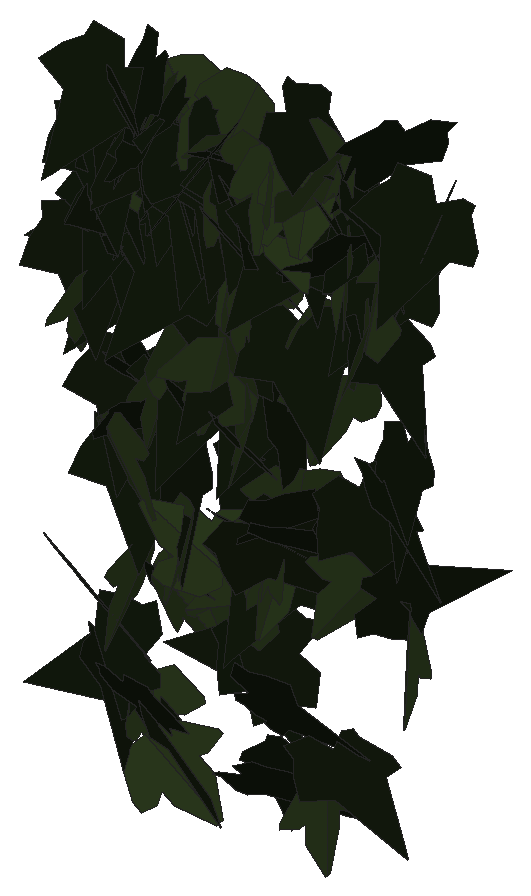
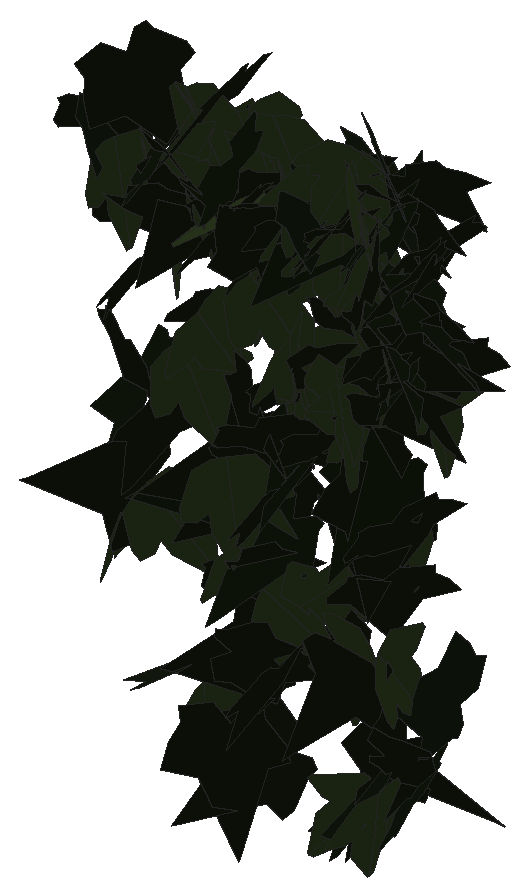
# SketchUp Ruby script. Lengths in inches.
U = 1.inch
M = Sketchup.active_model
def pt(a) = Geom::Point3d.new(a.map { |v| v * U })
def face(e, loops, mat)
  f = e.add_face(loops[0].map { |a| pt(a) })
  loops[1..].each { |l| e.add_face(l.map { |a| pt(a) }).erase! }
  f.material = f.back_material = mat if mat
  f
end
# faces: each face lists its corners as indices into pts; further lists are holes
def faces(e, pts, list, mat = nil) = list.each { |f| face(e, (f[0].is_a?(Array) ? f : [f]).map { |l| l.map { |i| pts[i] } }, mat) }
# xy, xz, yz: faces in a plane at the given z, y or x. An outline is a flat list of corners, or four numbers for a rectangle; further outlines are holes
def ring(l) = l.size == 4 ? [[l[0], l[1]], [l[2], l[1]], [l[2], l[3]], [l[0], l[3]]] : l.each_slice(2).to_a
def flat(e, list, mat, &to3) = list.each { |f| face(e, (f[0].is_a?(Array) ? f : [f]).map { |l| ring(l).map { |u, v| to3.(u, v) } }, mat) }
def xy(e, z, list, mat = nil) = flat(e, list, mat) { |x, y| [x, y, z] }
def xz(e, y, list, mat = nil) = flat(e, list, mat) { |x, z| [x, y, z] }
def yz(e, x, list, mat = nil) = flat(e, list, mat) { |y, z| [x, y, z] }
def lines(e, pts, list) = list.each { |a, b| e.add_line(pt(pts[a]), pt(pts[b])) }
# prism: a flat outline (further loops are holes) pulled along v
def prism(e, loops, v, mat = nil)
  f = face(e, loops, mat); d = Geom::Vector3d.new(v.map { |x| x * U })
  f.pushpull(f.normal.samedirection?(d) ? d.length : -d.length)
end
def box(e, o, s, mat = nil) = prism(e, [[o, [o[0] + s[0], o[1], o[2]], [o[0] + s[0], o[1] + s[1], o[2]], [o[0], o[1] + s[1], o[2]]]], [0, 0, s[2]], mat)
def at(x, y, z, deg = 0) = Geom::Transformation.translation(pt([x, y, z])) * Geom::Transformation.rotation(ORIGIN, Z_AXIS, deg.degrees)
def axes(o, x, y, z) = Geom::Transformation.new([*x, 0, *y, 0, *z, 0, *pt(o).to_a, 1])
def part(name) = M.definitions.add(name)
# library, detail: a bought-in or finely detailed component or shape, given as its bounding box
def library(name, o, s) = part(name).tap { |d| box(d.entities, o, s) }
def detail(e, o, s) = box(e.add_group.entities, o, s)
def put(e, d, t, mat = nil) = e.add_instance(d, t).tap { |i| i.material = mat if mat }
def group(e, t, mat = nil) = e.add_group.tap { |g| g.transformation = t; g.material = mat if mat }.entities
root = M.entities
M.materials.add("efeu1").color = [18, 25, 13]
M.materials.add("efeu2").color = [43, 57, 29]
c1 = part("ivyleaf_10")
p = [[0,0.5,-0.03],[-0.0625,2.02,-0.43],[-0.19,2.01,-0.46],[-0.54,1.05,-0.29],[-0.52,0.625,-0.18],[-0.83,0.76,-0.28],
  [-1.16,0.64,-0.33],[-1.15,0.33,-0.24],[-0.77,-0.39,0.02],[-0.3,-0.51,0.16],[0.04,-0.48,0.23],[-0.02,2.01,-0.4375],
  [-0.06,2.01,-0.43],[0.04,-0.49,0.23],[0.67,-0.49,0.14],[1.38,0.36,-0.2],[1.375,0.51,-0.24],[0.81,0.65,-0.19],
  [0.62,0.59,-0.15],[0.6,1.09,-0.28],[0.5,1.23,-0.31]]
faces(c1.entities,p,[[0,1,2,3,4,5,6,7,8,9,10],[11,12,0,13,14,15,16,17,18,19,20]],"efeu2")
c2 = part("ivyleaf_9")
p = [[1.54,2.16,1.25],[1.36,2.04,1.19],[-0.21,0.99,0.68],[-0.71,1.11,0.82],[-0.85,0.86,0.67],[-0.8,0.17,0.21],
  [-0.9,-0.01,0.1],[-0.67,-0.16,-0.02],[-0.08,-0.08,-0.05],[-0.03,-0.6,-0.4],[0.65,-0.88,-0.66],[0.83,-0.6,-0.49],
  [1.29,-0.42,-0.43],[1.8125,-0.07,-0.26],[1.21,0.44,0.15]]
faces(c2.entities,p,[[0,1,2,3,4,5,6,7,8,9,10,11,12,13,14]],"efeu1")
put(root,c1,axes([46.42,222.2,239.09],[-0.18687,-0.45242,0.10196],[0.01066,-0.11409,-0.48669],[0.46364,-0.17973,0.05229]))
put(root,c1,axes([48.57,222.03,240.14],[0.19422,-0.41581,-0.19845],[-0.07159,0.18551,-0.45876],[0.45514,0.20661,0.01252]))
put(root,c1,axes([47.91,222.2,234.14],[-0.01441,-0.49777,0.04491],[0.14775,-0.04716,-0.47534],[0.47745,-0.00043,0.14845]))
put(root,c2,axes([48.07,222.21,234.64],[0.17664,-0.46352,-0.06285],[0.1854,0.13106,-0.44548],[0.42945,0.13407,0.21817]))
put(root,c1,axes([47.25,222.21,241.76],[0.23344,0.42123,-0.13441],[-0.08511,-0.10634,-0.48109],[-0.43389,0.24749,0.02205]))
put(root,c2,axes([47.02,222.09,235.06],[0.41586,-0.08524,0.26419],[0.25869,-0.05361,-0.42451],[0.10069,0.48976,-0.00049]))
put(root,c2,axes([47.41,222.5,240.875],[-0.31856,-0.36533,0.12269],[-0.08262,-0.09074,-0.48471],[0.37642,-0.32909,-0.00255]))
put(root,c2,axes([47.125,221.98,237.26],[-0.04423,-0.06313,-0.49402],[0.1932,0.45496,-0.07543],[0.45904,-0.19756,-0.01585]))
put(root,c2,axes([44.83,222.46,241.98],[-0.41084,-0.28433,0.01913],[-0.00302,-0.02921,-0.49914],[0.28496,-0.41025,0.02228]))
put(root,c1,axes([46.875,222.07,238.46],[0.2035,-0.33058,-0.31513],[-0.16599,0.26787,-0.38819],[0.42548,0.26261,-0.00072]))
put(root,c1,axes([46.9375,222.19,241.64],[0.41646,-0.22108,-0.16639],[-0.12125,0.12446,-0.46884],[0.24872,0.43085,0.05006]))
put(root,c1,axes([45.87,222.27,236.7],[0.34721,-0.35866,-0.02838],[-0.00942,0.03036,-0.49899],[0.35966,0.34704,0.01432]))
put(root,c2,axes([45.65,221.98,241.66],[-0.16626,0.41848,0.21733],[-0.16013,0.16664,-0.44338],[-0.44353,-0.21703,0.07861]))
put(root,c2,axes([45.83,222.42,239.98],[-0.47455,-0.15731,-0.00731],[0.00761,0.00027,-0.49994],[0.15729,-0.47461,0.00214]))
put(root,c1,axes([48.63,222.18,240.17],[0.40084,-0.28958,0.07396],[-0.05901,0.04462,0.4945],[-0.29299,-0.40516,0.0016]))
put(root,c1,axes([44.57,222.27,239.35],[0.0171,-0.49805,-0.04069],[0.00491,0.04088,-0.4983],[0.49968,0.01664,0.00629]))
put(root,c1,axes([44.9,222.29,237.51],[-0.33765,0.2221,-0.29439],[0.25155,-0.15316,-0.40406],[-0.26966,-0.42097,-0.00831]))
put(root,c2,axes([47.24,221.97,237.3],[0.32648,0.13241,0.35479],[0.31842,0.15757,-0.35182],[-0.20498,0.45567,0.01856]))
put(root,c2,axes([46.6,222.63,240.59],[-0.02732,-0.24224,0.43654],[0.10822,-0.42968,-0.23166],[0.48738,0.08183,0.07591]))
put(root,c2,axes([45.21,222.1,234.53],[0.46391,0.06793,-0.17372],[-0.17364,-0.01278,-0.46871],[-0.06812,0.4952,0.01173]))
put(root,c2,axes([44.73,222.68,240.35],[-0.07226,-0.19063,0.45655],[-0.09926,-0.44643,-0.20211],[0.48469,-0.11984,0.02668]))
put(root,c2,axes([48.58,222.43,238.05],[0.29534,-0.38285,0.12727],[0.07739,-0.10104,-0.48353],[0.39596,0.30531,-0.00043]))
put(root,c2,axes([47.3,222.1,237.08],[0.40834,-0.06084,0.28206],[0.28835,0.10414,-0.39498],[-0.01068,0.48524,0.12014]))
put(root,c1,axes([48.93,222.48,236.27],[-0.13278,0.34249,-0.33922],[0.07943,-0.33149,-0.36579],[-0.47546,-0.15103,0.03362]))
put(root,c2,axes([44.22,222.4,235.53],[0.32861,-0.28889,0.24199],[0.19161,-0.14838,-0.43734],[0.3245,0.38016,0.01319]))
put(root,c1,axes([46.89,222.13,240.04],[-0.05069,0.47946,0.13248],[-0.02425,0.13062,-0.48203],[-0.49683,-0.0553,0.01001]))
put(root,c1,axes([46.97,222.31,236.84],[0.4392,-0.19955,-0.13145],[-0.10824,0.07909,-0.4817],[0.21304,0.45158,0.02627]))
put(root,c2,axes([44.55,222.48,241.1875],[0.02173,-0.49573,-0.06147],[0.02959,0.0627,-0.49517],[0.49865,0.01788,0.03207]))
put(root,c2,axes([45.24,222.5,238.07],[0.10524,-0.14329,0.46732],[0.32516,-0.33639,-0.17637],[0.36495,0.34104,0.02238]))
put(root,c1,axes([44.99,222.59,235.8],[0.11629,-0.39728,0.28044],[0.09858,-0.2631,-0.4136],[0.47619,0.15149,0.01714]))
put(root,c1,axes([45.5,222.47,238.5],[0.07603,-0.48302,0.10444],[0.03952,-0.09939,-0.48843],[0.4926,0.08253,0.02307]))
put(root,c2,axes([46.37,222.27,240.68],[0.45637,-0.20428,0.0008],[0.02021,0.04322,-0.49772],[0.20327,0.45432,0.04771]))
put(root,c2,axes([45.48,222.54,241.5],[-0.49125,-0.09,0.02399],[-0.02451,0.00067,-0.4994],[0.08986,-0.49183,-0.00507]))
put(root,c2,axes([47.375,222.48,239.6],[-0.1139,-0.44482,-0.1979],[0.09754,0.17828,-0.45684],[0.47698,-0.14268,0.04616]))
put(root,c2,axes([45.27,222.49,242.21],[-0.37767,0.10785,-0.30942],[0.30192,-0.06892,-0.39254],[-0.12732,-0.48334,-0.01306]))
put(root,c2,axes([45.17,222.73,241.25],[0.00783,-0.37095,0.33517],[0.06732,-0.33137,-0.36832],[0.49539,0.05089,0.04475]))
put(root,c2,axes([44.41,222.51,239.86],[-0.15924,-0.43992,-0.17638],[0.0508,0.16915,-0.46777],[0.47123,-0.16689,-0.00917]))
put(root,c1,axes([46.71,222.22,238.8],[-0.06522,0.04191,-0.49395],[-0.42133,0.25783,0.07751],[0.2612,0.42634,0.00168]))
put(root,c2,axes([46,222.65,240.91],[-0.20325,-0.45671,-0.01015],[-0.00088,0.01151,-0.49987],[0.45682,-0.20318,-0.00548]))
put(root,c2,axes([44.6,222.7,234.27],[0.11077,-0.40845,0.26626],[0.06247,-0.25891,-0.42316],[0.48356,0.12702,-0.00632]))
put(root,c2,axes([44.85,222.56,241.72],[-0.40211,-0.13511,-0.26467],[0.25918,0.05839,-0.42358],[0.14537,-0.47784,0.02307]))
put(root,c2,axes([45.9,222.3125,241.65],[0.03804,-0.33646,-0.3679],[0.02761,0.36982,-0.33536],[0.49779,0.0052,0.04672]))
put(root,c1,axes([45.57,222.23,233.75],[0.2526,0.27415,0.33322],[0.24011,0.23151,-0.37249],[-0.35852,0.3482,-0.01469]))
put(root,c1,axes([46.08,222.51,236.24],[0.19996,0.31079,0.33679],[-0.25218,-0.23219,0.36399],[0.38265,-0.31543,0.06389]))
put(root,c2,axes([46.46,222.12,238.29],[0.39437,0.13956,-0.27386],[-0.30533,0.12664,-0.37515],[-0.03535,0.46312,0.18511]))
put(root,c1,axes([47.82,222.58,240.69],[0.33802,-0.21424,0.29974],[0.2629,-0.14474,-0.39992],[0.25812,0.42796,0.0148]))
put(root,c2,axes([48.78,222.56,238.57],[-0.31296,-0.02809,-0.38893],[0.38933,0.00545,-0.31367],[0.02186,-0.49918,0.01846]))
put(root,c2,axes([46.38,222.75,239.06],[-0.23362,-0.41522,0.1517],[-0.0914,-0.1225,-0.47607],[0.43251,-0.25017,-0.01867]))
put(root,c1,axes([47.55,222.375,241.27],[-0.09202,-0.46118,0.16984],[0.11643,0.14742,0.46337],[-0.47747,0.12483,0.08026]))
put(root,c2,axes([44.81,222.61,240.5],[-0.42554,-0.18116,-0.18999],[0.18464,0.05069,-0.46189],[0.18661,-0.46326,0.02376]))
put(root,c2,axes([45.88,222.71,238.48],[-0.27179,-0.41898,0.02416],[-0.01314,-0.02028,-0.49942],[0.41947,-0.27211,0.00002]))
put(root,c1,axes([48.23,222.61,236.75],[-0.24207,-0.3143,0.30433],[-0.194,-0.23463,-0.39663],[0.39213,-0.31011,-0.00835]))
put(root,c2,axes([46.59,222.75,241.18],[-0.23194,-0.44293,-0.00376],[0.09622,-0.04624,-0.48847],[0.43237,-0.22732,0.10669]))
put(root,c2,axes([48.25,222.42,237.89],[0.07463,-0.39869,-0.29237],[-0.06361,0.28548,-0.40553],[0.49029,0.09773,-0.00811]))
put(root,c1,axes([47.48,222.49,241.625],[0.3215,0.37521,-0.07652],[-0.05772,-0.05128,-0.494],[-0.37856,0.32648,0.01034]))
put(root,c1,axes([46.68,222.5,235.9375],[-0.19165,0.01516,0.46156],[-0.45056,-0.11578,-0.18328],[0.10132,-0.48617,0.05804]))
put(root,c2,axes([49.02,222.72,241.61],[-0.35549,-0.34923,-0.04081],[0.02118,0.03666,-0.4982],[0.35097,-0.35594,-0.01127]))
put(root,c2,axes([46.27,222.74,241.07],[-0.18078,-0.46587,-0.01672],[0.00484,0.01606,-0.49972],[0.46615,-0.18084,-0.0013]))
put(root,c1,axes([47.24,222.23,240.81],[0.36,-0.31773,-0.13944],[0.29533,0.38606,-0.11722],[0.18215,0.00203,0.46563]))
put(root,c2,axes([46.82,222.22,233.92],[0.46952,0.12244,0.12065],[0.09161,0.11874,-0.47698],[-0.14546,0.47001,0.08907]))
put(root,c2,axes([45.29,222.62,234],[0.30549,-0.38469,0.09323],[0.06802,-0.06499,-0.49107],[0.38994,0.31272,0.01262]))
put(root,c2,axes([45,222.58,234.63],[-0.43368,0.06608,0.23991],[-0.23605,0.04337,-0.43864],[-0.07878,-0.49371,-0.00642]))
put(root,c2,axes([45.63,222.69,237.3],[-0.27302,-0.02533,-0.41811],[0.41863,-0.03384,-0.27131],[-0.01455,-0.49821,0.03968]))
put(root,c1,axes([46.32,222.45,240.93],[-0.02439,0.4994,0.00153],[0.00165,0.00161,-0.49999],[-0.4994,-0.02439,-0.00173]))
put(root,c1,axes([47.02,222.6875,236.62],[0.11342,0.40455,-0.27106],[-0.06753,-0.26256,-0.42012],[-0.48226,0.13191,-0.00492]))
put(root,c2,axes([47.05,222.73,235.3125],[-0.17522,-0.21573,-0.41564],[-0.27463,-0.31212,0.27778],[-0.37931,0.32564,-0.00911]))
put(root,c1,axes([45.42,222.625,235.73],[-0.20399,0.09811,-0.44583],[0.39477,-0.20729,-0.22624],[-0.22923,-0.4443,0.00711]))
put(root,c2,axes([47.32,222.34,242.34],[0.29613,-0.23255,-0.32898],[-0.13521,0.32724,-0.35303],[0.3795,0.29805,0.13092]))
put(root,c2,axes([47.34,222.39,238.55],[-0.07115,0.01387,-0.49472],[-0.49473,-0.01569,0.07071],[-0.01356,0.49956,0.01595]))
put(root,c2,axes([47.8,222.2,240.75],[0.29729,0.37822,0.13626],[0.08107,0.10959,-0.48106],[-0.39376,0.30812,0.00384]))
put(root,c2,axes([46.91,222.81,236.53],[-0.35711,-0.34995,0.00289],[-0.00351,-0.00055,-0.49999],[0.34995,-0.35712,-0.00206]))
put(root,c2,axes([45.73,222.83,241.04],[0.01792,-0.48822,0.1064],[0.02809,-0.10531,-0.48798],[0.49889,0.02346,0.02365]))
put(root,c1,axes([45.66,222.24,238.61],[0.04614,-0.22817,0.4425],[-0.07785,0.43562,0.23275],[-0.49174,-0.09038,0.00467]))
put(root,c1,axes([46.07,222.68,241.34],[-0.0758,-0.48288,0.10525],[-0.03522,-0.10093,-0.48844],[0.49296,-0.08146,-0.01872]))
put(root,c1,axes([45.32,222.61,241.33],[0.23826,-0.4377,-0.04061],[-0.02394,0.0332,-0.49832],[0.43893,0.23941,-0.00513]))
put(root,c2,axes([45.49,222.81,241.24],[-0.21877,-0.44732,-0.04517],[0.02235,0.03935,-0.49795],[0.44904,-0.21989,0.00278]))
put(root,c2,axes([49.13,222.68,241.52],[-0.31651,0.24627,-0.29862],[0.24566,-0.17029,-0.40081],[-0.29912,-0.40044,-0.01321]))
put(root,c2,axes([44.75,222.58,240.76],[-0.34749,0.3443,-0.10349],[0.03836,-0.1076,-0.48678],[-0.35746,-0.34624,0.04836]))
put(root,c2,axes([48.39,222.67,239.84],[0.17645,-0.45764,-0.09712],[-0.02102,0.09594,-0.49026],[0.46736,0.17709,0.01462]))
put(root,c2,axes([46.09,222.82,241.48],[-0.32376,0.19108,-0.32965],[0.18319,-0.30124,-0.35454],[-0.3341,-0.35035,0.12505]))
put(root,c1,axes([47.72,222.55,241.91],[0.39744,-0.10866,-0.28326],[-0.24218,0.16755,-0.40407],[0.18273,0.45839,0.08055]))
put(root,c2,axes([48.44,222.89,240.64],[-0.4028,-0.29622,0.00159],[0.01579,-0.02414,-0.49917],[0.29581,-0.40208,0.0288]))
put(root,c2,axes([46.64,222.34,236.9375],[0.46969,0.14154,-0.09674],[-0.13492,0.1311,-0.46326],[-0.10577,0.46128,0.16135]))
put(root,c2,axes([48.03,222.84,241.37],[0.21151,-0.43209,0.13623],[0.05622,-0.12415,-0.48107],[0.44956,0.21882,-0.00394]))
put(root,c2,axes([44.58,222.8125,240.9375],[0.11157,-0.48739,-0.00103],[0.00062,0.0012,-0.5],[0.48739,0.11157,0.00087]))
put(root,c2,axes([45.54,222.89,241.3],[0.07654,-0.48485,0.09521],[0.0004,-0.09628,-0.49064],[0.49411,0.07518,-0.01435]))
put(root,c2,axes([44.77,222.57,241.78],[0.41177,-0.24847,-0.13678],[-0.11696,0.07091,-0.48093],[0.2584,0.42806,0.00028]))
put(root,c2,axes([48.66,222.28,236.78],[0.11831,0.29416,-0.38661],[0.04979,0.38848,0.31082],[0.48324,-0.11205,0.06263]))
put(root,c1,axes([45.06,222.55,240.56],[0.24772,0.42496,0.08968],[0.02187,0.09091,-0.49118],[-0.43377,0.24728,0.02646]))
put(root,c1,axes([46.43,222.66,242.07],[0.46786,-0.06926,-0.16221],[-0.15524,0.05653,-0.47191],[0.08371,0.49194,0.0314]))
put(root,c1,axes([45.32,222.75,241.83],[0.17208,-0.46611,0.05592],[0.02308,-0.05109,-0.49685],[0.46889,0.17358,0.00393]))
put(root,c1,axes([46.65,222.79,240.01],[-0.31219,-0.26816,0.28395],[-0.18294,-0.22077,-0.40963],[0.34507,-0.35965,0.03973]))
put(root,c2,axes([46.65,222.85,240.47],[0.15805,0.14009,0.45321],[-0.38468,-0.24166,0.20885],[0.27756,-0.4147,0.03139]))
put(root,c1,axes([45.28,222.69,241.32],[0.4778,-0.13754,0.05279],[0.06345,0.03041,-0.49502],[0.13296,0.47975,0.04651]))
put(root,c2,axes([47.29,222.56,234.19],[0.27191,0.30039,-0.29297],[-0.20704,-0.2076,-0.40501],[-0.36497,0.34157,0.01149]))
put(root,c2,axes([48.14,222.55,241],[-0.30726,0.25866,0.29781],[-0.23365,0.1848,-0.40157],[-0.31781,-0.38593,0.0073]))
put(root,c1,axes([44.76,222.99,239.77],[-0.06486,0.07297,-0.49038],[0.21944,-0.43925,-0.09439],[-0.44457,-0.22746,0.02495]))
put(root,c1,axes([45.45,222.73,241.99],[-0.43521,-0.09575,-0.22678],[0.2442,-0.10994,-0.42223],[0.03099,-0.47828,0.14245]))
put(root,c2,axes([44.52,222.76,239.92],[0.33272,-0.37294,0.01464],[0.02823,0.00558,-0.49917],[0.37216,0.33299,0.02477]))
put(root,c1,axes([47.68,222.82,238.79],[-0.23323,-0.4111,0.16309],[-0.07564,-0.14458,-0.47262],[0.43575,-0.24514,0.00525]))
put(root,c2,axes([45.08,222.98,240.66],[0.03909,-0.09765,0.48881],[0.17725,-0.45554,-0.10518],[0.46589,0.18151,-0.001]))
put(root,c2,axes([46.46,222.77,237.59],[0.1861,-0.44194,-0.14161],[-0.0473,0.13372,-0.47946],[0.46166,0.19185,0.00796]))
put(root,c2,axes([48.55,222.77,242.35],[-0.06647,0.3579,-0.34276],[-0.0539,-0.349,-0.35397],[-0.49262,-0.01011,0.08498]))
put(root,c1,axes([47.16,222.75,237.47],[-0.35467,-0.34569,0.06861],[-0.04099,-0.05622,-0.49514],[0.35004,-0.35685,0.01154]))
put(root,c2,axes([46.54,223.01,238.46],[-0.33765,-0.36859,-0.01147],[0.06019,-0.03975,-0.49477],[0.36382,-0.3355,0.07122]))
put(root,c1,axes([48.69,222.76,240.99],[-0.10234,-0.48941,0.0012],[-0.002,-0.00081,-0.5],[0.48941,-0.10234,-0.00179]))
put(root,c2,axes([46.9375,222.88,241.54],[0.29744,-0.36339,0.17169],[0.11314,-0.12925,-0.46957],[0.38566,0.31818,0.00534]))
put(root,c1,axes([45.59,222.71,240.97],[0.21593,0.45081,-0.01198],[-0.00667,-0.01009,-0.49985],[-0.45092,0.21602,0.00166]))
put(root,c2,axes([44.9,222.96,239.94],[-0.09965,-0.15037,-0.46633],[-0.26017,-0.38701,0.18038],[-0.41519,0.2786,-0.00111]))
put(root,c2,axes([44.65,222.95,240.15],[-0.08862,-0.49022,-0.04278],[0.00417,0.04272,-0.49815],[0.49207,-0.08865,-0.00348]))
put(root,c1,axes([45.97,222.65,241.68],[0.14032,0.47692,0.05345],[0.02289,0.04897,-0.49707],[-0.47936,0.14195,-0.00809]))
put(root,c1,axes([46.26,222.83,239.48],[-0.04444,0.4544,-0.20384],[0.0062,-0.20413,-0.45639],[-0.49798,-0.04309,0.01251]))
put(root,c2,axes([45.14,222.5,237.91],[0.13663,0.47992,-0.0318],[-0.01587,-0.02854,-0.49893],[-0.48071,0.13735,0.00744]))
put(root,c2,axes([46.45,222.78,235.32],[0.17428,-0.42777,-0.19141],[-0.0546,0.18429,-0.46158],[0.46545,0.18179,0.01752]))
put(root,c2,axes([44.8,222.94,237.1],[-0.20434,-0.43162,-0.14816],[0.10467,0.11368,-0.47552],[0.44417,-0.22535,0.0439]))
put(root,c2,axes([45.8,222.44,241.2],[0.42953,0.24646,0.06898],[-0.00219,0.1383,-0.48049],[-0.25592,0.41247,0.11989]))
put(root,c2,axes([45.05,222.51,238.26],[0.44551,0.17328,-0.14661],[-0.17502,0.05663,-0.46493],[-0.14452,0.46558,0.11111]))
put(root,c1,axes([47.37,222.92,239.48],[0.09891,0.41352,-0.2631],[-0.12576,-0.238,-0.42135],[-0.47371,0.14953,0.05693]))
put(root,c2,axes([45.375,222.62,235.74],[0.49559,0.02586,-0.06105],[-0.06095,-0.00339,-0.49626],[-0.02608,0.49932,-0.0002]))
put(root,c1,axes([45.07,222.88,241.13],[-0.07051,0.44722,-0.21219],[0.0072,-0.21338,-0.45213],[-0.49495,-0.06681,0.02365]))
put(root,c1,axes([45.53,222.78,239.27],[0.49432,-0.0737,-0.0146],[-0.00162,0.08672,-0.49242],[0.07512,0.48688,0.08549]))
put(root,c2,axes([44.6,223.03,237.9375],[-0.1228,-0.48443,-0.01575],[0.00262,0.01559,-0.49975],[0.48468,-0.12282,-0.00129]))
put(root,c1,axes([45.07,222.78,234.08],[0.04158,0.49536,-0.05373],[-0.00648,-0.05338,-0.4971],[-0.49823,0.04204,0.00198]))
put(root,c2,axes([44.95,222.5,240.06],[-0.12888,0.40705,0.26019],[-0.11366,0.23618,-0.42579],[-0.46954,-0.1689,0.03165]))
put(root,c2,axes([44.74,223.03,239.46],[-0.43595,-0.24394,0.02093],[-0.0208,-0.00568,-0.49953],[0.24395,-0.43642,-0.0052]))
put(root,c2,axes([47.02,223.03,240.87],[0.07836,-0.4907,0.05542],[0.00861,-0.05475,-0.49692],[0.49375,0.07884,-0.00013]))
